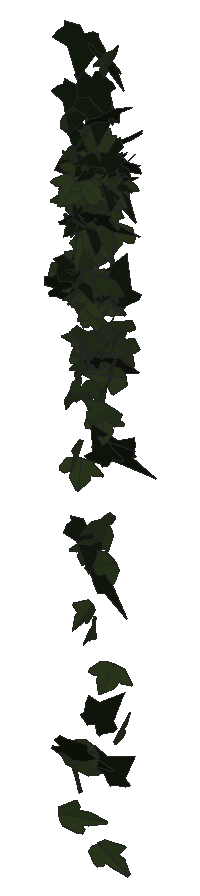
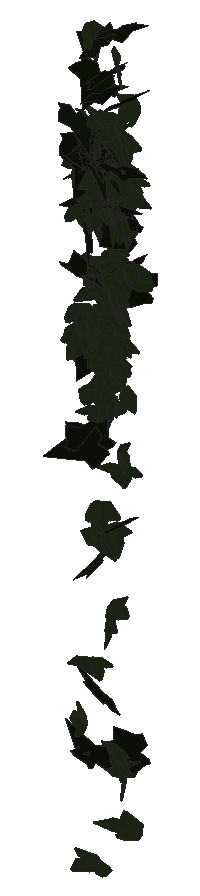
# SketchUp Ruby script. Lengths in inches.
U = 1.inch
M = Sketchup.active_model
def pt(a) = Geom::Point3d.new(a.map { |v| v * U })
def face(e, loops, mat)
  f = e.add_face(loops[0].map { |a| pt(a) })
  loops[1..].each { |l| e.add_face(l.map { |a| pt(a) }).erase! }
  f.material = f.back_material = mat if mat
  f
end
# faces: each face lists its corners as indices into pts; further lists are holes
def faces(e, pts, list, mat = nil) = list.each { |f| face(e, (f[0].is_a?(Array) ? f : [f]).map { |l| l.map { |i| pts[i] } }, mat) }
# xy, xz, yz: faces in a plane at the given z, y or x. An outline is a flat list of corners, or four numbers for a rectangle; further outlines are holes
def ring(l) = l.size == 4 ? [[l[0], l[1]], [l[2], l[1]], [l[2], l[3]], [l[0], l[3]]] : l.each_slice(2).to_a
def flat(e, list, mat, &to3) = list.each { |f| face(e, (f[0].is_a?(Array) ? f : [f]).map { |l| ring(l).map { |u, v| to3.(u, v) } }, mat) }
def xy(e, z, list, mat = nil) = flat(e, list, mat) { |x, y| [x, y, z] }
def xz(e, y, list, mat = nil) = flat(e, list, mat) { |x, z| [x, y, z] }
def yz(e, x, list, mat = nil) = flat(e, list, mat) { |y, z| [x, y, z] }
def lines(e, pts, list) = list.each { |a, b| e.add_line(pt(pts[a]), pt(pts[b])) }
# prism: a flat outline (further loops are holes) pulled along v
def prism(e, loops, v, mat = nil)
  f = face(e, loops, mat); d = Geom::Vector3d.new(v.map { |x| x * U })
  f.pushpull(f.normal.samedirection?(d) ? d.length : -d.length)
end
def box(e, o, s, mat = nil) = prism(e, [[o, [o[0] + s[0], o[1], o[2]], [o[0] + s[0], o[1] + s[1], o[2]], [o[0], o[1] + s[1], o[2]]]], [0, 0, s[2]], mat)
def at(x, y, z, deg = 0) = Geom::Transformation.translation(pt([x, y, z])) * Geom::Transformation.rotation(ORIGIN, Z_AXIS, deg.degrees)
def axes(o, x, y, z) = Geom::Transformation.new([*x, 0, *y, 0, *z, 0, *pt(o).to_a, 1])
def part(name) = M.definitions.add(name)
# library, detail: a bought-in or finely detailed component or shape, given as its bounding box
def library(name, o, s) = part(name).tap { |d| box(d.entities, o, s) }
def detail(e, o, s) = box(e.add_group.entities, o, s)
def put(e, d, t, mat = nil) = e.add_instance(d, t).tap { |i| i.material = mat if mat }
def group(e, t, mat = nil) = e.add_group.tap { |g| g.transformation = t; g.material = mat if mat }.entities
root = M.entities
M.materials.add("1026 AP 7946 SUNNY SIDE UP").color = [254, 231, 186]
M.materials.add("efeu1").color = [18, 25, 13]
M.materials.add("efeu2").color = [43, 57, 29]
c1 = part("ivyleaf_10")
p = [[0,0.5,-0.03],[-0.0625,2.02,-0.43],[-0.19,2.01,-0.46],[-0.54,1.05,-0.29],[-0.52,0.625,-0.18],[-0.83,0.76,-0.28],
  [-1.16,0.64,-0.33],[-1.15,0.33,-0.24],[-0.77,-0.39,0.02],[-0.3,-0.51,0.16],[0.04,-0.48,0.23],[-0.02,2.01,-0.4375],
  [-0.06,2.01,-0.43],[0.04,-0.49,0.23],[0.67,-0.49,0.14],[1.38,0.36,-0.2],[1.375,0.51,-0.24],[0.81,0.65,-0.19],
  [0.62,0.59,-0.15],[0.6,1.09,-0.28],[0.5,1.23,-0.31]]
faces(c1.entities,p,[[0,1,2,3,4,5,6,7,8,9,10],[11,12,0,13,14,15,16,17,18,19,20]],"efeu2")
c2 = part("ivyleaf_9")
p = [[1.54,2.16,1.25],[1.36,2.04,1.19],[-0.21,0.99,0.68],[-0.71,1.11,0.82],[-0.85,0.86,0.67],[-0.8,0.17,0.21],
  [-0.9,-0.01,0.1],[-0.67,-0.16,-0.02],[-0.08,-0.08,-0.05],[-0.03,-0.6,-0.4],[0.65,-0.88,-0.66],[0.83,-0.6,-0.49],
  [1.29,-0.42,-0.43],[1.8125,-0.07,-0.26],[1.21,0.44,0.15]]
faces(c2.entities,p,[[0,1,2,3,4,5,6,7,8,9,10,11,12,13,14]],"efeu1")
put(root,c1,axes([108.99,212.68,260.37],[-0.03094,-0.12467,-0.20598],[0.0887,0.19158,-0.12812],[0.35875,-0.05812,0.01391]),"1026 AP 7946 SUNNY SIDE UP")
put(root,c1,axes([108.75,212.6,262.76],[0.03239,0.03453,0.24875],[0.31048,0.13957,-0.03713],[-0.22464,0.19788,-0.01545]),"1026 AP 7946 SUNNY SIDE UP")
put(root,c1,axes([108.97,212.85,263.79],[0.17635,-0.2061,0.03555],[0.08511,-0.01051,-0.23787],[0.31768,0.11722,0.04399]),"1026 AP 7946 SUNNY SIDE UP")
put(root,c1,axes([109.11,212.89,262.91],[-0.18837,-0.19041,0.06982],[-0.03544,-0.06696,-0.23157],[0.3164,-0.12087,0.01563]),"1026 AP 7946 SUNNY SIDE UP")
put(root,c1,axes([109.04,212.93,262.37],[0.13339,-0.21289,-0.01549],[0.02379,0.02085,-0.2349],[0.33461,0.08339,0.02288]),"1026 AP 7946 SUNNY SIDE UP")
put(root,c1,axes([109.05,212.49,266.13],[0.10568,0.06655,0.2409],[-0.09088,0.23967,-0.05184],[-0.37075,-0.03977,0.08138]),"1026 AP 7946 SUNNY SIDE UP")
put(root,c1,axes([109.05,212.93,261.14],[-0.23573,0.16406,-0.00248],[-0.01792,-0.01492,-0.22825],[-0.2574,-0.14921,0.01816]),"1026 AP 7946 SUNNY SIDE UP")
put(root,c1,axes([109.3,212.84,263.55],[-0.20775,0.03693,-0.19948],[-0.29222,0.05513,0.14164],[0.1043,0.22801,-0.00049]),"1026 AP 7946 SUNNY SIDE UP")
put(root,c1,axes([109.07,212.67,264.39],[-0.31654,-0.12524,-0.0199],[0.05434,-0.02073,-0.24157],[0.19152,-0.2011,0.03565]),"1026 AP 7946 SUNNY SIDE UP")
put(root,c1,axes([109.1,212.95,263.99],[-0.28326,0.1518,0.03324],[-0.05763,0.00507,-0.24182],[-0.23683,-0.18279,0.01909]),"1026 AP 7946 SUNNY SIDE UP")
put(root,c2,axes([108.79,212.5,262.53],[0.16126,0.04166,0.24828],[0.36382,0.06736,-0.11315],[-0.12348,0.25288,-0.00913]),"1026 AP 7946 SUNNY SIDE UP")
put(root,c1,axes([109.08,212.68,265.46],[-0.03983,-0.24131,-0.06198],[0.03414,0.05672,-0.24914],[0.38905,-0.02968,0.01552]),"1026 AP 7946 SUNNY SIDE UP")
put(root,c1,axes([109.08,212.9375,267.31],[0.17711,-0.22636,-0.04024],[0.00329,0.0431,-0.25933],[0.36083,0.11071,0.02212]),"1026 AP 7946 SUNNY SIDE UP")
put(root,c1,axes([109.02,213.01,261.0625],[0.21576,0.16538,0.04237],[-0.00463,0.05392,-0.21792],[-0.26757,0.13242,0.03793]),"1026 AP 7946 SUNNY SIDE UP")
put(root,c1,axes([109.04,212.82,259.2],[0.08202,-0.17268,0.13092],[0.08461,-0.1171,-0.18592],[0.32728,0.07355,0.01526]),"1026 AP 7946 SUNNY SIDE UP")
put(root,c1,axes([109.125,212.62,252.59],[-0.16742,0.17917,0.07251],[-0.08689,0.0474,-0.21322],[-0.28934,-0.1179,0.02208]),"1026 AP 7946 SUNNY SIDE UP")
put(root,c1,axes([109.11,212.68,264.02],[0.1715,-0.21992,-0.0603],[-0.02104,0.05722,-0.2522],[0.35672,0.10911,0.01411]),"1026 AP 7946 SUNNY SIDE UP")
put(root,c1,axes([109.11,212.88,260.98],[-0.00531,-0.22396,0.02065],[0.00393,-0.02135,-0.23086],[0.35373,-0.00313,0.00287]),"1026 AP 7946 SUNNY SIDE UP")
put(root,c1,axes([109.12,212.89,263.92],[-0.36307,0.07003,0.00312],[-0.01551,-0.02352,-0.24733],[-0.10909,-0.22972,0.02479]),"1026 AP 7946 SUNNY SIDE UP")
put(root,c2,axes([109.03,212.85,266.39],[-0.12334,-0.23214,0.09279],[-0.02,-0.09196,-0.25241],[0.39178,-0.07778,0.01633]),"1026 AP 7946 SUNNY SIDE UP")
put(root,c1,axes([109.16,212.77,261.41],[-0.30693,0.0927,0.05163],[-0.08496,0.00126,-0.22151],[-0.1418,-0.2014,0.02095]),"1026 AP 7946 SUNNY SIDE UP")
put(root,c1,axes([109.1,212.79,263.01],[0.23235,-0.18184,0.00489],[-0.01037,-0.01279,-0.24107],[0.28588,0.14732,-0.01272]),"1026 AP 7946 SUNNY SIDE UP")
put(root,c1,axes([109.125,212.62,264.72],[0.35525,0.0339,-0.07802],[-0.11208,-0.03422,-0.23445],[-0.06732,0.23587,-0.02136]),"1026 AP 7946 SUNNY SIDE UP")
put(root,c1,axes([109.21,212.82,262.38],[0.2498,-0.12751,-0.12624],[-0.14551,0.07928,-0.20937],[0.23604,0.18382,0.00453]),"1026 AP 7946 SUNNY SIDE UP")
put(root,c1,axes([108.97,212.91,263.07],[-0.27694,-0.09045,-0.12868],[0.23356,-0.05096,-0.17878],[0.06275,-0.20952,0.09751]),"1026 AP 7946 SUNNY SIDE UP")
put(root,c1,axes([109.15,212.93,261.22],[-0.0856,0.21359,0.03442],[-0.09257,0.01728,-0.22051],[-0.32679,-0.06085,0.05344]),"1026 AP 7946 SUNNY SIDE UP")
put(root,c1,axes([109.1,212.86,262.68],[-0.18274,0.19895,-0.0268],[-0.00499,-0.03317,-0.23672],[-0.31569,-0.11464,0.01925]),"1026 AP 7946 SUNNY SIDE UP")
put(root,c1,axes([109.16,212.96,262.49],[0.17192,-0.2006,-0.02959],[-0.02453,0.02291,-0.23521],[0.31744,0.11041,-0.00215]),"1026 AP 7946 SUNNY SIDE UP")
put(root,c2,axes([108.99,212.66,263.05],[0.0769,-0.21647,-0.10711],[-0.01345,0.10321,-0.22762],[0.37653,0.0479,0.01374]),"1026 AP 7946 SUNNY SIDE UP")
put(root,c1,axes([108.9,212.69,251.59],[-0.04074,0.00909,0.24359],[0.28133,0.15635,0.01492],[-0.24338,0.1792,-0.02352]),"1026 AP 7946 SUNNY SIDE UP")
put(root,c1,axes([109.19,212.8,261.46],[-0.34195,-0.04819,0.01971],[-0.01277,-0.05097,-0.22442],[0.08069,-0.2123,0.04802]),"1026 AP 7946 SUNNY SIDE UP")
put(root,c1,axes([109.13,212.93,260.16],[-0.13663,0.19985,0.00386],[-0.01442,-0.00114,-0.22432],[-0.31394,-0.08692,0.00863]),"1026 AP 7946 SUNNY SIDE UP")
put(root,c1,axes([109.17,212.94,264.81],[0.02387,-0.23618,-0.05501],[0.0266,0.05306,-0.24265],[0.37935,0.01114,0.02047]),"1026 AP 7946 SUNNY SIDE UP")
put(root,c1,axes([109.17,212.89,260.27],[-0.23372,0.15725,0.01065],[-0.02787,-0.00379,-0.22237],[-0.24614,-0.14889,0.01507]),"1026 AP 7946 SUNNY SIDE UP")
put(root,c1,axes([109.1,212.75,258.88],[0.31814,0.09283,-0.00054],[0.00911,-0.01514,-0.22881],[-0.14569,0.20176,-0.01548]),"1026 AP 7946 SUNNY SIDE UP")
put(root,c1,axes([109.3,212.67,264.95],[0.33946,-0.04484,-0.14026],[-0.21665,0.00133,-0.22593],[0.0608,0.2551,-0.02194]),"1026 AP 7946 SUNNY SIDE UP")
put(root,c2,axes([109.11,212.9,265.04],[-0.20625,-0.18377,-0.10272],[0.11455,0.06885,-0.23148],[0.30732,-0.14899,0.01734]),"1026 AP 7946 SUNNY SIDE UP")
put(root,c1,axes([109.24,212.71,262.49],[-0.12592,-0.21843,0.00674],[-0.00379,-0.00741,-0.23972],[0.34366,-0.08012,-0.00017]),"1026 AP 7946 SUNNY SIDE UP")
put(root,c1,axes([109.22,212.86,262.37],[0.11526,-0.21803,-0.00264],[-0.00148,0.00108,-0.23696],[0.34283,0.07331,-0.00013]),"1026 AP 7946 SUNNY SIDE UP")
put(root,c1,axes([109.23,212.97,261.16],[-0.22325,-0.16814,-0.01417],[0.02562,0.00297,-0.22643],[0.2639,-0.14252,0.01]),"1026 AP 7946 SUNNY SIDE UP")
put(root,c2,axes([108.93,212.77,263.74],[0.24313,0.17889,-0.11075],[0.09275,0.09219,0.24369],[0.31565,-0.16488,0.0137]),"1026 AP 7946 SUNNY SIDE UP")
put(root,c1,axes([109.23,212.7,265.76],[0.15062,-0.23946,0.03791],[0.00324,-0.04022,-0.2656],[0.38127,0.09494,-0.01272]),"1026 AP 7946 SUNNY SIDE UP")
put(root,c1,axes([109.14,212.82,263.35],[-0.0533,-0.13526,0.19526],[0.14142,-0.18502,-0.12006],[0.33879,0.05595,0.08084]),"1026 AP 7946 SUNNY SIDE UP")
put(root,c1,axes([109.23,212.91,264.22],[0.09186,-0.23385,0.0106],[0.00267,-0.01156,-0.24838],[0.36815,0.05844,-0.00085]),"1026 AP 7946 SUNNY SIDE UP")
put(root,c2,axes([109.3,212.9,264.19],[-0.33588,-0.1147,0.00678],[0.00562,-0.02188,-0.24897],[0.18062,-0.21261,0.02034]),"1026 AP 7946 SUNNY SIDE UP")
put(root,c1,axes([109.27,212.72,262.71],[0.04243,0.16486,-0.17094],[-0.13029,-0.15043,-0.1678],[-0.34506,0.07708,0.04234]),"1026 AP 7946 SUNNY SIDE UP")
put(root,c1,axes([109.14,212.7,252.71],[-0.2996,-0.06125,0.0956],[0.1359,0.03532,0.20628],[-0.1107,0.20912,-0.00548]),"1026 AP 7946 SUNNY SIDE UP")
put(root,c2,axes([108.92,212.53,253.09],[0.3317,0.00244,0.14422],[0.21866,-0.03291,-0.2155],[0.02545,0.25102,-0.02816]),"1026 AP 7946 SUNNY SIDE UP")
put(root,c2,axes([109.07,212.74,265.76],[0.20147,-0.1884,-0.11265],[-0.06213,0.1034,-0.23291],[0.33598,0.13209,0.02448]),"1026 AP 7946 SUNNY SIDE UP")
put(root,c1,axes([109.26,212.98,261.48],[-0.04583,-0.22004,-0.00446],[0.04633,-0.00082,-0.22667],[0.34291,-0.0293,0.03003]),"1026 AP 7946 SUNNY SIDE UP")
put(root,c1,axes([109.23,212.9,264.43],[0.2561,-0.18073,-0.00233],[0.03013,0.01892,-0.24899],[0.28258,0.16178,0.02866]),"1026 AP 7946 SUNNY SIDE UP")
put(root,c1,axes([109.36,212.75,265.64],[0.32403,-0.02152,-0.13195],[-0.17958,0.0839,-0.20353],[0.09683,0.2276,0.06408]),"1026 AP 7946 SUNNY SIDE UP")
put(root,c2,axes([109.2,212.74,267.76],[-0.14458,-0.24221,0.00167],[0.00985,-0.00558,-0.26681],[0.38076,-0.09183,0.00753]),"1026 AP 7946 SUNNY SIDE UP")
put(root,c1,axes([109.36,212.7,253.09],[0.25492,-0.1063,-0.11224],[-0.15654,0.04519,-0.19888],[0.18016,0.18969,-0.01399]),"1026 AP 7946 SUNNY SIDE UP")
put(root,c1,axes([109.28,212.76,255.96],[-0.04689,-0.1314,0.1825],[0.04583,-0.18028,-0.1332],[0.34473,0.00609,0.04253]),"1026 AP 7946 SUNNY SIDE UP")
put(root,c1,axes([109.31,212.82,263.14],[-0.06884,-0.22954,-0.03065],[0.01335,0.02734,-0.24055],[0.36345,-0.04448,0.00303]),"1026 AP 7946 SUNNY SIDE UP")
put(root,c1,axes([109.23,212.97,261.31],[0.23099,0.16144,-0.01044],[-0.00103,-0.01433,-0.22475],[-0.25444,0.14662,-0.00857]),"1026 AP 7946 SUNNY SIDE UP")
put(root,c1,axes([109.375,212.85,262.57],[0.23836,-0.13465,-0.11675],[-0.0952,0.09948,-0.20601],[0.25901,0.16047,0.03172]),"1026 AP 7946 SUNNY SIDE UP")
put(root,c2,axes([109.16,212.89,264.13],[0.07069,-0.23787,0.00617],[0.01036,-0.00623,-0.24937],[0.37406,0.04512,0.00574]),"1026 AP 7946 SUNNY SIDE UP")
put(root,c2,axes([109.48,212.91,264.85],[-0.03796,0.1827,0.16622],[-0.03893,0.15842,-0.1889],[-0.3802,-0.03446,0.00274]),"1026 AP 7946 SUNNY SIDE UP")
put(root,c1,axes([109.38,212.91,264],[-0.16419,-0.21032,0.04976],[-0.00395,-0.05379,-0.24123],[0.33972,-0.10228,0.02125]),"1026 AP 7946 SUNNY SIDE UP")
put(root,c1,axes([109.375,212.61,261.18],[0.04225,-0.17377,-0.16391],[-0.01545,0.15818,-0.17988],[0.36911,0.02651,0.01123]),"1026 AP 7946 SUNNY SIDE UP")
put(root,c1,axes([109.39,212.85,261.55],[-0.06545,0.17777,0.13458],[-0.11054,0.11427,-0.18402],[-0.32781,-0.07402,0.03518]),"1026 AP 7946 SUNNY SIDE UP")
put(root,c1,axes([109.37,212.6,261.7],[-0.33315,0.06981,-0.00687],[0.00014,-0.02219,-0.22892],[-0.11033,-0.21083,0.02044]),"1026 AP 7946 SUNNY SIDE UP")
put(root,c1,axes([109.28,212.86,261.46],[0.33348,0.06848,0.02217],[0.03161,0.00652,-0.22955],[-0.10817,0.21303,0.00128]),"1026 AP 7946 SUNNY SIDE UP")
put(root,c1,axes([109.4,212.67,265.6],[0.32534,-0.12073,-0.07633],[-0.07493,0.06292,-0.2446],[0.20915,0.21033,0.0311]),"1026 AP 7946 SUNNY SIDE UP")
put(root,c1,axes([109.4,212.73,255.64],[0.03989,-0.18453,-0.12691],[0.01911,0.12391,-0.18954],[0.34743,0.01437,0.02499]),"1026 AP 7946 SUNNY SIDE UP")
put(root,c1,axes([109.43,212.625,257.43],[-0.09414,-0.22547,0.02464],[-0.00039,-0.026,-0.24039],[0.35674,-0.05953,0.00624]),"1026 AP 7946 SUNNY SIDE UP")
put(root,c2,axes([109.57,212.75,265.02],[-0.13611,0.22425,0.03974],[-0.04161,0.02971,-0.24705],[-0.35502,-0.08945,0.01372]),"1026 AP 7946 SUNNY SIDE UP")
put(root,c2,axes([109.3,212.74,257.6],[-0.04959,-0.25526,0.03989],[0.00031,-0.04049,-0.26515],[0.40631,-0.03112,0.00507]),"1026 AP 7946 SUNNY SIDE UP")
put(root,c1,axes([109.39,212.875,260.61],[-0.16417,-0.18507,-0.05208],[0.07759,0.0285,-0.2168],[0.29107,-0.11198,0.02842]),"1026 AP 7946 SUNNY SIDE UP")
put(root,c1,axes([109.57,212.66,263.65],[0.1734,-0.12407,-0.17782],[-0.21345,0.10751,-0.16902],[0.25605,0.17365,-0.02048]),"1026 AP 7946 SUNNY SIDE UP")
put(root,c1,axes([109.46,212.89,264.32],[-0.03562,-0.24033,0.02317],[0.00022,-0.02397,-0.24882],[0.37976,-0.02253,0.00232]),"1026 AP 7946 SUNNY SIDE UP")
put(root,c1,axes([109.37,212.93,261.17],[0.32884,-0.1079,0.05261],[0.05629,-0.04287,-0.2417],[0.1795,0.21112,-0.02059]),"1026 AP 7946 SUNNY SIDE UP")
put(root,c1,axes([109.5,212.77,262.4],[0.23162,0.13153,-0.12538],[-0.15491,-0.07331,-0.20365],[-0.23633,0.17697,0.01061]),"1026 AP 7946 SUNNY SIDE UP")
put(root,c1,axes([109.41,212.77,262.85],[-0.22429,-0.17906,-0.08592],[0.11107,0.04851,-0.23431],[0.28934,-0.15742,0.02333]),"1026 AP 7946 SUNNY SIDE UP")
put(root,c1,axes([109.57,212.65,265.69],[0.34268,-0.02201,0.12974],[-0.18848,0.05203,0.22316],[-0.07043,-0.24633,0.03403]),"1026 AP 7946 SUNNY SIDE UP")
put(root,c1,axes([109.51,212.73,262.85],[-0.38221,-0.01712,-0.008],[0.01456,-0.02291,-0.25],[0.02564,-0.24211,0.02279]),"1026 AP 7946 SUNNY SIDE UP")
put(root,c1,axes([109.35,212.79,264.58],[0.08984,-0.19468,0.13013],[0.20327,-0.08253,-0.1901],[0.30418,0.11265,0.0886]),"1026 AP 7946 SUNNY SIDE UP")
put(root,c2,axes([109.7,212.46,265.3],[-0.09233,0.21968,0.09999],[-0.08923,0.0831,-0.23162],[-0.36613,-0.07565,0.03123]),"1026 AP 7946 SUNNY SIDE UP")
put(root,c1,axes([109.46,212.87,264.24],[-0.35357,-0.05294,-0.06624],[0.1101,-0.02148,-0.23527],[0.07024,-0.2328,0.03532]),"1026 AP 7946 SUNNY SIDE UP")
put(root,c1,axes([109.54,212.77,265.29],[-0.02781,-0.24356,0.04563],[0.01022,-0.04624,-0.25165],[0.38952,-0.01618,0.00986]),"1026 AP 7946 SUNNY SIDE UP")
put(root,c2,axes([109.41,212.83,264.07],[-0.04786,-0.24035,0.03446],[-0.00462,-0.03472,-0.24978],[0.38184,-0.03055,0.00129]),"1026 AP 7946 SUNNY SIDE UP")
put(root,c1,axes([109.27,212.84,262.04],[0.22212,0.00208,0.18823],[0.28709,-0.01023,-0.14537],[0.01073,0.23071,-0.00679]),"1026 AP 7946 SUNNY SIDE UP")
put(root,c2,axes([109.37,212.8,266.87],[0.06047,-0.23824,-0.08672],[-0.00452,0.08337,-0.24792],[0.39658,0.03728,0.0104]),"1026 AP 7946 SUNNY SIDE UP")
put(root,c2,axes([109.38,212.84,265.14],[0.0061,-0.24441,-0.05318],[0.02184,0.05037,-0.25109],[0.39173,0.001,0.01483]),"1026 AP 7946 SUNNY SIDE UP")
put(root,c1,axes([109.55,212.91,264.6875],[0.05447,-0.04852,0.26325],[-0.10994,0.24686,0.05943],[-0.39437,-0.07551,0.01979]),"1026 AP 7946 SUNNY SIDE UP")
put(root,c1,axes([109.58,212.93,261.8],[0.01004,-0.22633,0.00226],[-0.00329,-0.00354,-0.23327],[0.35591,0.00635,-0.00222]),"1026 AP 7946 SUNNY SIDE UP")
put(root,c1,axes([109.59,212.9,264.58],[-0.0711,-0.23759,0.03131],[-0.00378,-0.03185,-0.24932],[0.37689,-0.04514,0.00341]),"1026 AP 7946 SUNNY SIDE UP")
put(root,c1,axes([109.6,212.86,264.41],[-0.13725,-0.22392,0.01601],[0.00514,-0.0193,-0.24749],[0.35305,-0.08677,0.00983]),"1026 AP 7946 SUNNY SIDE UP")
put(root,c2,axes([109.49,212.82,266.41],[-0.08463,-0.24693,0.01038],[-0.00303,-0.01133,-0.26042],[0.38868,-0.05386,0.00023]),"1026 AP 7946 SUNNY SIDE UP")
put(root,c1,axes([109.53,213.01,261.46],[0.18172,-0.15801,0.10474],[0.07764,-0.09071,-0.20182],[0.28586,0.12509,-0.01177]),"1026 AP 7946 SUNNY SIDE UP")
put(root,c1,axes([109.55,212.94,261.29],[-0.05627,0.2163,0.01847],[-0.01359,0.01549,-0.22568],[-0.34085,-0.03633,0.00595]),"1026 AP 7946 SUNNY SIDE UP")
put(root,c1,axes([109.75,212.73,260.23],[-0.25399,-0.07628,0.14072],[-0.16932,-0.08906,-0.18237],[0.17927,-0.19219,0.02711]),"1026 AP 7946 SUNNY SIDE UP")
put(root,c1,axes([109.625,212.84,264.04],[-0.05879,-0.22708,0.08193],[-0.00097,-0.0817,-0.23724],[0.379,-0.03543,0.0121]),"1026 AP 7946 SUNNY SIDE UP")
put(root,c1,axes([109.6,212.74,257.875],[-0.1258,-0.23826,-0.07816],[0.0487,0.06817,-0.25841],[0.3895,-0.08548,0.00706]),"1026 AP 7946 SUNNY SIDE UP")
put(root,c1,axes([109.67,212.83,257.62],[0.21706,-0.17576,-0.07034],[-0.08302,0.04391,-0.22955],[0.28404,0.14715,-0.01334]),"1026 AP 7946 SUNNY SIDE UP")
put(root,c1,axes([109.64,212.92,261.49],[0.05578,-0.22001,0.03345],[-0.00754,-0.0349,-0.22954],[0.3499,0.03432,-0.01028]),"1026 AP 7946 SUNNY SIDE UP")
put(root,c1,axes([109.47,212.68,265.45],[0.37975,0.04304,-0.09416],[0.13429,0.04072,0.2518],[0.0855,-0.25509,0.02274]),"1026 AP 7946 SUNNY SIDE UP")
put(root,c1,axes([109.54,212.82,259.96],[0.22575,0.16373,0.0049],[0.02272,-0.00759,-0.22378],[-0.25651,0.14342,-0.01551]),"1026 AP 7946 SUNNY SIDE UP")
put(root,c1,axes([109.39,213.07,250.9],[0.21149,0.07328,0.18257],[0.26604,0.05549,-0.15596],[-0.14067,0.21511,-0.02047]),"1026 AP 7946 SUNNY SIDE UP")
put(root,c1,axes([109.7,212.875,261.66],[-0.33634,-0.05036,0.02645],[-0.03072,-0.0296,-0.22519],[0.08362,-0.21343,0.02365]),"1026 AP 7946 SUNNY SIDE UP")
put(root,c1,axes([109.61,212.94,261.74],[0.23096,-0.16445,0.05084],[0.0547,-0.03635,-0.22736],[0.26481,0.15094,0.00262]),"1026 AP 7946 SUNNY SIDE UP")
put(root,c2,axes([109.74,212.9,259.2],[0.1795,0.09471,0.22645],[-0.33765,-0.06572,0.14403],[0.16445,-0.23831,0.04855]),"1026 AP 7946 SUNNY SIDE UP")
put(root,c1,axes([109.9,212.8125,260.94],[0.08426,-0.00739,-0.22513],[-0.34105,-0.02994,-0.05394],[-0.043,0.22297,-0.01337]),"1026 AP 7946 SUNNY SIDE UP")
put(root,c1,axes([109.52,212.72,262.38],[0.11342,0.08428,0.21144],[0.139,0.18649,-0.11007],[-0.31923,0.11115,0.0272]),"1026 AP 7946 SUNNY SIDE UP")
put(root,c1,axes([109.74,212.83,264.31],[-0.10468,-0.23206,0.04633],[-0.0007,-0.04796,-0.24865],[0.37207,-0.06538,0.01257]),"1026 AP 7946 SUNNY SIDE UP")
put(root,c2,axes([109.85,212.85,265.32],[0.12557,0.18903,-0.13884],[-0.17753,-0.09414,-0.20388],[-0.32008,0.12637,0.05861]),"1026 AP 7946 SUNNY SIDE UP")
put(root,c2,axes([109.86,212.76,263.49],[-0.01294,0.00285,-0.26701],[-0.34119,0.14179,0.00953],[0.22298,0.21713,-0.00091]),"1026 AP 7946 SUNNY SIDE UP")
put(root,c2,axes([109.47,212.92,267.42],[0.10439,-0.21694,0.1425],[0.11305,-0.12283,-0.23266],[0.38952,0.09379,0.02934]),"1026 AP 7946 SUNNY SIDE UP")
put(root,c1,axes([109.7,212.81,262.84],[-0.31856,0.11165,-0.04064],[0.03609,-0.04093,-0.23722],[-0.183,-0.20243,0.02396]),"1026 AP 7946 SUNNY SIDE UP")
put(root,c2,axes([109.45,212.55,264.13],[0.30883,0.04283,0.15082],[0.2263,0.02586,-0.20689],[-0.07837,0.24345,-0.00308]),"1026 AP 7946 SUNNY SIDE UP")
put(root,c2,axes([109.89,212.75,265.32],[-0.17917,0.2158,-0.01898],[-0.00097,-0.02252,-0.25128],[-0.34073,-0.11342,0.0107]),"1026 AP 7946 SUNNY SIDE UP")
put(root,c1,axes([109.89,212.59,257.19],[0.23157,-0.06442,-0.16673],[-0.23265,0.06467,-0.16522],[0.14353,0.20876,0.00119]),"1026 AP 7946 SUNNY SIDE UP")
put(root,c1,axes([109.77,212.96,261.8125],[-0.04314,-0.22267,0.02406],[0.00082,-0.02487,-0.23125],[0.35226,-0.02721,0.00349]),"1026 AP 7946 SUNNY SIDE UP")
put(root,c2,axes([109.67,212.74,261.22],[0.34161,0.11692,-0.05511],[-0.05751,-0.04585,-0.25337],[-0.19428,0.21916,-0.0219]),"1026 AP 7946 SUNNY SIDE UP")
put(root,c1,axes([109.72,212.87,254.81],[0.31362,0.08892,-0.0539],[-0.06286,-0.03956,-0.22432],[-0.14999,0.2025,-0.0187]),"1026 AP 7946 SUNNY SIDE UP")
put(root,c1,axes([109.78,212.79,267.55],[-0.0082,-0.25848,0.00175],[0.00925,-0.00329,-0.26629],[0.40636,-0.00514,0.0061]),"1026 AP 7946 SUNNY SIDE UP")
put(root,c2,axes([109.72,212.73,264.86],[0.19499,0.22594,0.06564],[0.06368,0.04892,-0.26496],[-0.36304,0.12993,-0.01122]),"1026 AP 7946 SUNNY SIDE UP")
put(root,c2,axes([109.75,212.7,264.9],[-0.11182,0.2192,-0.13157],[-0.09776,0.11486,0.23712],[0.38777,0.09217,0.02184]),"1026 AP 7946 SUNNY SIDE UP")
put(root,c1,axes([109.8,212.72,260.89],[0.11292,-0.20811,-0.00943],[-0.01947,0.00415,-0.22652],[0.32689,0.07214,-0.01023]),"1026 AP 7946 SUNNY SIDE UP")
put(root,c1,axes([109.53,212.64,263.85],[0.25275,-0.00396,0.19797],[0.30044,-0.02426,-0.16528],[0.03324,0.24938,-0.01146]),"1026 AP 7946 SUNNY SIDE UP")
put(root,c2,axes([109.78,212.8,262.57],[-0.35695,0.07429,0.13098],[0.20304,-0.01026,0.24445],[0.11011,0.25978,-0.02615]),"1026 AP 7946 SUNNY SIDE UP")
put(root,c2,axes([109.61,212.6875,256.83],[0.21581,-0.21579,-0.05948],[-0.04751,0.04776,-0.26318],[0.34752,0.14053,0.00095]),"1026 AP 7946 SUNNY SIDE UP")
put(root,c1,axes([109.84,212.89,263.93],[-0.30319,-0.1333,0.05583],[0.01778,-0.10546,-0.22329],[0.22601,-0.17052,0.09246]),"1026 AP 7946 SUNNY SIDE UP")
put(root,c2,axes([109.68,212.53,253.88],[-0.17273,0.17576,0.15878],[0.15013,-0.1205,0.21235],[0.33438,0.1449,-0.01332]),"1026 AP 7946 SUNNY SIDE UP")
put(root,c2,axes([110.04,212.6,265.67],[-0.34918,0.0993,0.03416],[-0.06262,-0.00964,-0.24935],[-0.15193,-0.22424,0.02428]),"1026 AP 7946 SUNNY SIDE UP")
put(root,c1,axes([109.77,212.9,264.89],[-0.3578,-0.06284,-0.06327],[0.10631,-0.01783,-0.24075],[0.08765,-0.23492,0.03371]),"1026 AP 7946 SUNNY SIDE UP")
put(root,c1,axes([109.84,212.875,261.25],[0.0919,-0.215,0.00304],[-0.00518,-0.00522,-0.22951],[0.33809,0.05836,-0.00434]),"1026 AP 7946 SUNNY SIDE UP")
put(root,c1,axes([109.85,212.68,263.71],[0.25081,-0.18347,-0.02923],[-0.0306,0.0193,-0.25033],[0.29006,0.16068,-0.00113]),"1026 AP 7946 SUNNY SIDE UP")
put(root,c1,axes([109.85,213.01,261.74],[0.07049,-0.2103,0.05667],[0.00444,-0.05681,-0.22166],[0.34225,0.04405,-0.00879]),"1026 AP 7946 SUNNY SIDE UP")
put(root,c1,axes([109.87,212.97,261.92],[-0.17482,-0.19562,0.00227],[0.01465,-0.0091,-0.23149],[0.30729,-0.11085,0.01233]),"1026 AP 7946 SUNNY SIDE UP")
put(root,c2,axes([109.57,212.93,259.29],[0.38645,0.01258,0.097],[0.14915,-0.02307,-0.25223],[-0.00542,0.26215,-0.02531]),"1026 AP 7946 SUNNY SIDE UP")
put(root,c1,axes([109.8,213.01,261.41],[-0.23873,-0.13441,-0.0906],[0.12158,0.04372,-0.2079],[0.22063,-0.16953,0.01654]),"1026 AP 7946 SUNNY SIDE UP")
put(root,c2,axes([109.77,212.88,265.06],[-0.07942,-0.23696,0.04783],[0.00086,-0.04892,-0.24965],[0.38009,-0.0494,0.01056]),"1026 AP 7946 SUNNY SIDE UP")
put(root,c2,axes([109.79,212.97,265.38],[-0.09424,-0.16186,0.17608],[0.007,-0.17803,-0.17221],[0.37113,-0.03775,0.04796]),"1026 AP 7946 SUNNY SIDE UP")
put(root,c1,axes([109.75,212.65,264.625],[-0.27754,0.08401,-0.15337],[0.16212,-0.11919,-0.1953],[-0.21522,-0.19813,0.05067]),"1026 AP 7946 SUNNY SIDE UP")
put(root,c1,axes([109.92,212.65,265.26],[0.26592,-0.16852,-0.07751],[-0.06948,0.06077,-0.24532],[0.28112,0.17443,0.01269]),"1026 AP 7946 SUNNY SIDE UP")
put(root,c2,axes([110.03,212.87,265.79],[-0.02906,0.24295,0.03596],[-0.05694,0.03055,-0.24845],[-0.3814,-0.02307,0.03435]),"1026 AP 7946 SUNNY SIDE UP")
put(root,c2,axes([109.89,212.41,266.48],[0.16008,0.22608,0.076],[0.03482,0.06949,-0.25489],[-0.37169,0.10388,0.00885]),"1026 AP 7946 SUNNY SIDE UP")
put(root,c1,axes([109.89,212.88,253.5],[0.1144,-0.14145,0.17429],[-0.08818,0.1613,0.16394],[-0.33636,-0.09039,0.0163]),"1026 AP 7946 SUNNY SIDE UP")
put(root,c1,axes([109.68,212.51,264.93],[0.17782,0.14452,0.19906],[0.17962,0.15487,-0.1881],[-0.33302,0.1607,0.00483]),"1026 AP 7946 SUNNY SIDE UP")
put(root,c1,axes([109.91,213.02,261.52],[-0.15037,-0.19918,0.00237],[0.03848,-0.01553,-0.22577],[0.31086,-0.09443,0.02909]),"1026 AP 7946 SUNNY SIDE UP")
put(root,c2,axes([109.71,212.76,252.75],[-0.12462,0.05198,0.23093],[0.25436,-0.15559,0.09531],[0.2567,0.17941,0.01767]),"1026 AP 7946 SUNNY SIDE UP")
put(root,c2,axes([109.74,212.88,264.9],[0.12727,-0.22319,-0.05537],[0.00544,0.05683,-0.24319],[0.36047,0.07795,0.02322]),"1026 AP 7946 SUNNY SIDE UP")
